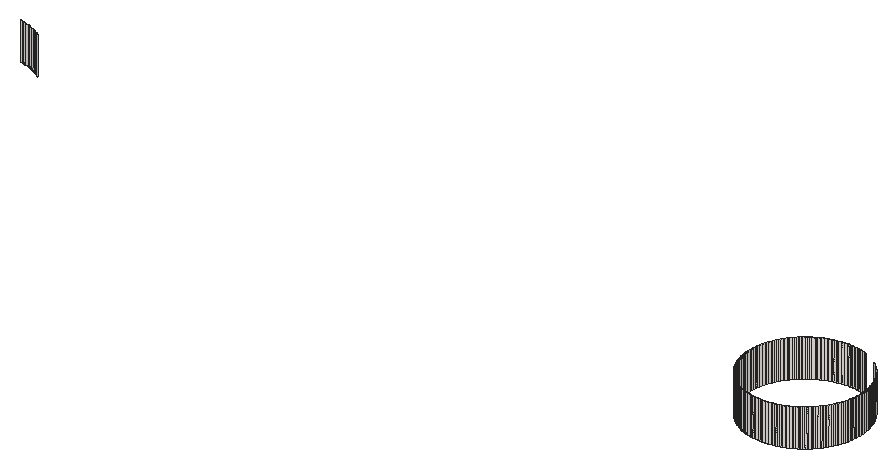
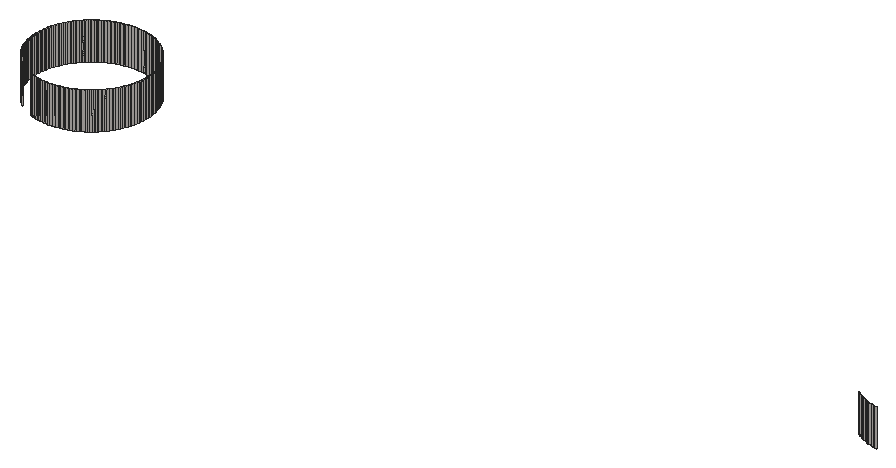
# SketchUp Ruby script. Lengths in inches.
U = 1.inch
M = Sketchup.active_model
def pt(a) = Geom::Point3d.new(a.map { |v| v * U })
def face(e, loops, mat)
  f = e.add_face(loops[0].map { |a| pt(a) })
  loops[1..].each { |l| e.add_face(l.map { |a| pt(a) }).erase! }
  f.material = f.back_material = mat if mat
  f
end
# faces: each face lists its corners as indices into pts; further lists are holes
def faces(e, pts, list, mat = nil) = list.each { |f| face(e, (f[0].is_a?(Array) ? f : [f]).map { |l| l.map { |i| pts[i] } }, mat) }
# xy, xz, yz: faces in a plane at the given z, y or x. An outline is a flat list of corners, or four numbers for a rectangle; further outlines are holes
def ring(l) = l.size == 4 ? [[l[0], l[1]], [l[2], l[1]], [l[2], l[3]], [l[0], l[3]]] : l.each_slice(2).to_a
def flat(e, list, mat, &to3) = list.each { |f| face(e, (f[0].is_a?(Array) ? f : [f]).map { |l| ring(l).map { |u, v| to3.(u, v) } }, mat) }
def xy(e, z, list, mat = nil) = flat(e, list, mat) { |x, y| [x, y, z] }
def xz(e, y, list, mat = nil) = flat(e, list, mat) { |x, z| [x, y, z] }
def yz(e, x, list, mat = nil) = flat(e, list, mat) { |y, z| [x, y, z] }
def lines(e, pts, list) = list.each { |a, b| e.add_line(pt(pts[a]), pt(pts[b])) }
# prism: a flat outline (further loops are holes) pulled along v
def prism(e, loops, v, mat = nil)
  f = face(e, loops, mat); d = Geom::Vector3d.new(v.map { |x| x * U })
  f.pushpull(f.normal.samedirection?(d) ? d.length : -d.length)
end
def box(e, o, s, mat = nil) = prism(e, [[o, [o[0] + s[0], o[1], o[2]], [o[0] + s[0], o[1] + s[1], o[2]], [o[0], o[1] + s[1], o[2]]]], [0, 0, s[2]], mat)
def at(x, y, z, deg = 0) = Geom::Transformation.translation(pt([x, y, z])) * Geom::Transformation.rotation(ORIGIN, Z_AXIS, deg.degrees)
def axes(o, x, y, z) = Geom::Transformation.new([*x, 0, *y, 0, *z, 0, *pt(o).to_a, 1])
def part(name) = M.definitions.add(name)
# library, detail: a bought-in or finely detailed component or shape, given as its bounding box
def library(name, o, s) = part(name).tap { |d| box(d.entities, o, s) }
def detail(e, o, s) = box(e.add_group.entities, o, s)
def put(e, d, t, mat = nil) = e.add_instance(d, t).tap { |i| i.material = mat if mat }
def group(e, t, mat = nil) = e.add_group.tap { |g| g.transformation = t; g.material = mat if mat }.entities
root = M.entities
M.materials.add("0001 AP 9436 AIR BREEZE").color = [243, 237, 232]
xz(root,40.5,[[68.91,106,68.98,108],[68.98,106,69.0625,108],[69.0625,106,69.14,108]],"0001 AP 9436 AIR BREEZE")
xz(root,40.51,[[68.75,106,68.83,108],[69.22,106,69.3,108]],"0001 AP 9436 AIR BREEZE")
xz(root,46.49,[[68.7,106,68.78,108],[69.17,106,69.25,108]],"0001 AP 9436 AIR BREEZE")
xz(root,46.5,[[68.86,106,68.9375,108],[68.9375,106,69.02,108],[69.02,106,69.09,108]],"0001 AP 9436 AIR BREEZE")
yz(root,66,[[43.36,106,43.4375,108],[43.4375,106,43.52,108],[43.52,106,43.59,108]],"0001 AP 9436 AIR BREEZE")
yz(root,66.01,[[43.2,106,43.28,108],[43.67,106,43.75,108]],"0001 AP 9436 AIR BREEZE")
yz(root,71.99,[[43.25,106,43.33,108],[43.72,106,43.8,108]],"0001 AP 9436 AIR BREEZE")
yz(root,72,[[43.41,106,43.48,108],[43.48,106,43.5625,108],[43.5625,106,43.64,108]],"0001 AP 9436 AIR BREEZE")
p = [[68.51,40.54,106],[68.4375,40.55,106],[68.4375,40.55,108],[68.51,40.54,108],[68.59,40.53,106],[68.59,40.53,108],
  [68.67,40.52,106],[68.67,40.52,108],[68.75,40.51,106],[68.75,40.51,108],[68.91,40.5,106],[68.83,40.51,106],
  [68.83,40.51,108],[68.91,40.5,108],[69.22,40.51,106],[69.14,40.5,106],[69.14,40.5,108],[69.22,40.51,108],
  [69.375,40.52,106],[69.3,40.51,106],[69.3,40.51,108],[69.375,40.52,108],[69.45,40.53,106],[69.45,40.53,108],
  [69.61,40.5625,106],[69.53,40.55,106],[69.53,40.55,108],[69.61,40.5625,108],[68.21,40.61,106],[68.13,40.63,106],
  [68.13,40.63,108],[68.21,40.61,108],[68.06,40.65,106],[68.06,40.65,108],[68.28,40.59,106],[68.28,40.59,108],
  [68.36,40.57,106],[68.36,40.57,108],[69.68,40.58,106],[69.68,40.58,108],[69.76,40.6,106],[69.76,40.6,108],
  [69.91,40.64,106],[69.84,40.62,106],[69.84,40.62,108],[69.91,40.64,108],[69.99,40.67,106],[69.99,40.67,108],
  [67.91,40.71,106],[67.84,40.73,106],[67.84,40.73,108],[67.91,40.71,108],[67.76,40.77,106],[67.76,40.77,108],
  [67.98,40.68,106],[67.98,40.68,108],[70.06,40.69,106],[70.06,40.69,108],[70.21,40.75,106],[70.13,40.72,106],
  [70.13,40.72,108],[70.21,40.75,108],[67.69,40.8,106],[67.625,40.83,106],[67.625,40.83,108],[67.69,40.8,108],
  [67.55,40.87,106],[67.55,40.87,108],[70.28,40.79,106],[70.28,40.79,108],[70.42,40.86,106],[70.35,40.82,106],
  [70.35,40.82,108],[70.42,40.86,108],[67.49,40.91,106],[67.42,40.95,106],[67.42,40.95,108],[67.49,40.91,108],
  [70.49,40.89,106],[70.49,40.89,108],[70.55,40.93,106],[70.55,40.93,108],[70.62,40.98,106],[70.62,40.98,108],
  [67.29,41.04,106],[67.22,41.08,106],[67.22,41.08,108],[67.29,41.04,108],[67.35,40.99,106],[67.35,40.99,108],
  [70.6875,41.02,106],[70.6875,41.02,108],[70.75,41.0625,106],[70.75,41.0625,108],[67.16,41.13,106],[67.1,41.18,106],
  [67.1,41.18,108],[67.16,41.13,108],[70.875,41.16,106],[70.8125,41.11,106],[70.8125,41.11,108],[70.875,41.16,108],
  [67.04,41.23,106],[67.04,41.23,108],[66.98,41.28,106],[66.98,41.28,108],[71,41.26,106],[70.9375,41.21,106],
  [70.9375,41.21,108],[71,41.26,108],[66.92,41.34,106],[66.92,41.34,108],[66.87,41.39,106],[66.87,41.39,108],
  [71.05,41.3125,106],[71.05,41.3125,108],[71.11,41.37,106],[71.11,41.37,108],[66.8125,41.45,106],[66.8125,41.45,108],
  [66.76,41.5,106],[66.76,41.5,108],[71.16,41.42,106],[71.16,41.42,108],[71.22,41.48,106],[71.22,41.48,108],
  [66.71,41.5625,106],[66.71,41.5625,108],[71.27,41.54,106],[71.27,41.54,108],[71.32,41.6,106],[71.32,41.6,108],
  [66.66,41.625,106],[66.61,41.6875,106],[66.61,41.6875,108],[66.66,41.625,108],[71.37,41.66,106],[71.37,41.66,108],
  [66.5625,41.75,106],[66.52,41.8125,106],[66.52,41.8125,108],[66.5625,41.75,108],[71.46,41.79,106],[71.42,41.72,106],
  [71.42,41.72,108],[71.46,41.79,108],[66.48,41.88,106],[66.48,41.88,108],[71.51,41.85,106],[71.51,41.85,108],
  [66.43,41.95,106],[66.43,41.95,108],[66.39,42.01,106],[66.39,42.01,108],[71.59,41.99,106],[71.55,41.92,106],
  [71.55,41.92,108],[71.59,41.99,108],[66.36,42.08,106],[66.36,42.08,108],[71.63,42.05,106],[71.63,42.05,108],
  [66.32,42.15,106],[66.32,42.15,108],[71.67,42.125,106],[71.67,42.125,108],[71.7,42.19,106],[71.7,42.19,108],
  [66.29,42.22,106],[66.29,42.22,108],[66.25,42.29,106],[66.25,42.29,108],[71.73,42.26,106],[71.73,42.26,108],
  [66.22,42.37,106],[66.22,42.37,108],[71.77,42.34,106],[71.77,42.34,108],[71.79,42.41,106],[71.79,42.41,108],
  [66.19,42.44,106],[66.19,42.44,108],[66.17,42.51,106],[66.17,42.51,108],[71.82,42.48,106],[71.82,42.48,108],
  [66.14,42.59,106],[66.14,42.59,108],[71.85,42.56,106],[71.85,42.56,108],[66.12,42.66,106],[66.12,42.66,108],
  [71.87,42.63,106],[71.87,42.63,108],[71.89,42.71,106],[71.89,42.71,108],[66.1,42.74,106],[66.1,42.74,108],
  [66.08,42.82,106],[66.08,42.82,108],[71.91,42.78,106],[71.91,42.78,108],[66.0625,42.89,106],[66.0625,42.89,108],
  [71.93,42.86,106],[71.93,42.86,108],[66.05,42.97,106],[66.05,42.97,108],[71.96,43.01,106],[71.95,42.9375,106],
  [71.95,42.9375,108],[71.96,43.01,108],[66.03,43.05,106],[66.03,43.05,108],[66.02,43.125,106],[66.02,43.125,108],
  [71.97,43.09,106],[71.97,43.09,108],[66.01,43.2,106],[66.01,43.2,108],[71.98,43.17,106],[71.98,43.17,108],
  [71.99,43.25,106],[71.99,43.25,108],[66.01,43.28,106],[66,43.36,106],[66,43.36,108],[66.01,43.28,108],
  [72,43.41,106],[71.99,43.33,106],[71.99,43.33,108],[72,43.41,108],[66,43.59,106],[66.01,43.67,106],
  [66.01,43.67,108],[66,43.59,108],[71.99,43.72,106],[72,43.64,106],[72,43.64,108],[71.99,43.72,108],
  [66.01,43.75,106],[66.02,43.83,106],[66.02,43.83,108],[66.01,43.75,108],[66.03,43.91,106],[66.03,43.91,108],
  [71.98,43.875,106],[71.99,43.8,106],[71.99,43.8,108],[71.98,43.875,108],[66.04,43.99,106],[66.04,43.99,108],
  [71.97,43.95,106],[71.97,43.95,108],[66.05,44.0625,106],[66.05,44.0625,108],[71.9375,44.11,106],[71.95,44.03,106],
  [71.95,44.03,108],[71.9375,44.11,108],[66.07,44.14,106],[66.07,44.14,108],[66.09,44.22,106],[66.09,44.22,108],
  [71.92,44.18,106],[71.92,44.18,108],[66.11,44.29,106],[66.11,44.29,108],[71.9,44.26,106],[71.9,44.26,108],
  [66.13,44.37,106],[66.13,44.37,108],[71.86,44.41,106],[71.88,44.34,106],[71.88,44.34,108],[71.86,44.41,108],
  [66.15,44.44,106],[66.15,44.44,108],[66.18,44.52,106],[66.18,44.52,108],[71.83,44.49,106],[71.83,44.49,108],
  [66.21,44.59,106],[66.21,44.59,108],[71.81,44.56,106],[71.81,44.56,108],[66.23,44.66,106],[66.23,44.66,108],
  [71.75,44.71,106],[71.78,44.63,106],[71.78,44.63,108],[71.75,44.71,108],[66.27,44.74,106],[66.27,44.74,108],
  [66.3,44.81,106],[66.3,44.81,108],[71.71,44.78,106],[71.71,44.78,108],[66.33,44.875,106],[66.33,44.875,108],
  [71.64,44.92,106],[71.68,44.85,106],[71.68,44.85,108],[71.64,44.92,108],[66.37,44.95,106],[66.37,44.95,108],
  [66.41,45.01,106],[66.41,45.01,108],[71.61,44.99,106],[71.61,44.99,108],[66.45,45.08,106],[66.45,45.08,108],
  [71.57,45.05,106],[71.57,45.05,108],[66.49,45.15,106],[66.49,45.15,108],[66.54,45.21,106],[66.54,45.21,108],
  [71.48,45.1875,106],[71.52,45.12,106],[71.52,45.12,108],[71.48,45.1875,108],[66.58,45.28,106],[66.58,45.28,108],
  [71.4375,45.25,106],[71.4375,45.25,108],[66.63,45.34,106],[66.63,45.34,108],[66.68,45.4,106],[66.68,45.4,108],
  [71.34,45.375,106],[71.39,45.3125,106],[71.39,45.3125,108],[71.34,45.375,108],[66.73,45.46,106],[66.73,45.46,108],
  [71.24,45.5,106],[71.29,45.4375,106],[71.29,45.4375,108],[71.24,45.5,108],[66.78,45.52,106],[66.78,45.52,108],
  [66.84,45.58,106],[66.84,45.58,108],[71.1875,45.55,106],[71.1875,45.55,108],[66.89,45.63,106],[66.89,45.63,108],
  [66.95,45.6875,106],[66.95,45.6875,108],[71.08,45.66,106],[71.13,45.61,106],[71.13,45.61,108],[71.08,45.66,108],
  [67,45.74,106],[67,45.74,108],[67.0625,45.79,106],[67.0625,45.79,108],[70.96,45.77,106],[71.02,45.72,106],
  [71.02,45.72,108],[70.96,45.77,108],[67.125,45.84,106],[67.125,45.84,108],[67.1875,45.89,106],[67.1875,45.89,108],
  [70.84,45.87,106],[70.9,45.82,106],[70.9,45.82,108],[70.84,45.87,108],[25.71,45.96,106],[25.78,45.92,106],
  [25.78,45.92,108],[25.71,45.96,108],[67.25,45.9375,106],[67.25,45.9375,108],[67.3125,45.98,106],[67.3125,45.98,108],
  [70.78,45.92,106],[70.78,45.92,108],[25.51,46.09,106],[25.58,46.05,106],[25.58,46.05,108],[25.51,46.09,108],
  [25.65,46.01,106],[25.65,46.01,108],[67.38,46.02,106],[67.38,46.02,108],[67.45,46.07,106],[67.45,46.07,108],
  [25.375,46.17,106],[25.45,46.13,106],[25.45,46.13,108],[25.375,46.17,108],[67.51,46.11,106],[67.51,46.11,108],
  [67.58,46.14,106],[67.58,46.14,108],[67.65,46.18,106],[67.65,46.18,108],[25.16,46.27,106],[25.24,46.23,106],
  [25.24,46.23,108],[25.16,46.27,108],[25.31,46.2,106],[25.31,46.2,108],[67.72,46.21,106],[67.72,46.21,108],
  [67.79,46.25,106],[67.79,46.25,108],[67.87,46.28,106],[67.87,46.28,108],[24.87,46.37,106],[24.94,46.35,106],
  [24.94,46.35,108],[24.87,46.37,108],[25.02,46.32,106],[25.02,46.32,108],[25.09,46.29,106],[25.09,46.29,108],
  [67.94,46.31,106],[67.94,46.31,108],[68.01,46.33,106],[68.01,46.33,108],[68.09,46.36,106],[68.09,46.36,108],
  [69.87,46.37,106],[69.94,46.35,106],[69.94,46.35,108],[69.87,46.37,108],[70.02,46.32,106],[70.02,46.32,108],
  [24.49,46.46,106],[24.5625,46.45,106],[24.5625,46.45,108],[24.49,46.46,108],[24.64,46.43,106],[24.64,46.43,108],
  [24.72,46.41,106],[24.72,46.41,108],[24.79,46.39,106],[24.79,46.39,108],[68.16,46.38,106],[68.16,46.38,108],
  [68.24,46.4,106],[68.24,46.4,108],[68.32,46.42,106],[68.32,46.42,108],[68.39,46.4375,106],[68.39,46.4375,108],
  [68.47,46.45,106],[68.47,46.45,108],[69.49,46.46,106],[69.5625,46.45,106],[69.5625,46.45,108],[69.49,46.46,108],
  [69.64,46.43,106],[69.64,46.43,108],[69.72,46.41,106],[69.72,46.41,108],[69.79,46.39,106],[69.79,46.39,108],
  [24.41,46.47,106],[24.41,46.47,108],[68.55,46.47,106],[68.55,46.47,108],[68.625,46.48,106],[68.625,46.48,108],
  [68.7,46.49,106],[68.7,46.49,108],[68.78,46.49,106],[68.86,46.5,106],[68.86,46.5,108],[68.78,46.49,108],
  [69.09,46.5,106],[69.17,46.49,106],[69.17,46.49,108],[69.09,46.5,108],[69.25,46.49,106],[69.33,46.48,106],
  [69.33,46.48,108],[69.25,46.49,108],[69.41,46.47,106],[69.41,46.47,108]]
faces(root,p,[[0,1,2,3],[4,0,3,5],[6,4,5,7],[8,6,7,9],[10,11,12,13],[14,15,16,17],[18,19,20,21],[22,18,21,23],
  [24,25,26,27],[25,22,23,26],[28,29,30,31],[29,32,33,30],[34,28,31,35],[36,34,35,37],[1,36,37,2],[38,24,27,39],
  [40,38,39,41],[42,43,44,45],[43,40,41,44],[46,42,45,47],[48,49,50,51],[49,52,53,50],[54,48,51,55],[32,54,55,33],
  [56,46,47,57],[58,59,60,61],[59,56,57,60],[62,63,64,65],[63,66,67,64],[52,62,65,53],[68,58,61,69],[70,71,72,73],
  [71,68,69,72],[74,75,76,77],[66,74,77,67],[78,70,73,79],[80,78,79,81],[82,80,81,83],[84,85,86,87],[88,84,87,89],
  [75,88,89,76],[90,82,83,91],[92,90,91,93],[94,95,96,97],[85,94,97,86],[98,99,100,101],[99,92,93,100],[95,102,103,96],
  [102,104,105,103],[106,107,108,109],[107,98,101,108],[104,110,111,105],[110,112,113,111],[114,106,109,115],[116,114,115,117],[112,118,119,113],
  [118,120,121,119],[122,116,117,123],[124,122,123,125],[120,126,127,121],[128,124,125,129],[130,128,129,131],[132,133,134,135],[126,132,135,127],
  [136,130,131,137],[138,139,140,141],[133,138,141,134],[142,143,144,145],[143,136,137,144],[139,146,147,140],[148,142,145,149],[146,150,151,147],
  [150,152,153,151],[154,155,156,157],[155,148,149,156],[152,158,159,153],[160,154,157,161],[158,162,163,159],[164,160,161,165],[166,164,165,167],
  [162,168,169,163],[168,170,171,169],[172,166,167,173],[170,174,175,171],[176,172,173,177],[178,176,177,179],[174,180,181,175],[180,182,183,181],
  [184,178,179,185],[182,186,187,183],[188,184,185,189],[186,190,191,187],[192,188,189,193],[194,192,193,195],[190,196,197,191],[196,198,199,197],
  [200,194,195,201],[198,202,203,199],[204,200,201,205],[202,206,207,203],[208,209,210,211],[209,204,205,210],[206,212,213,207],[212,214,215,213],
  [216,208,211,217],[214,218,219,215],[220,216,217,221],[222,220,221,223],[224,225,226,227],[228,229,230,231],[232,233,234,235],[236,237,238,239],
  [240,241,242,243],[241,244,245,242],[246,247,248,249],[244,250,251,245],[252,246,249,253],[250,254,255,251],[256,257,258,259],[257,252,253,258],
  [254,260,261,255],[260,262,263,261],[264,256,259,265],[262,266,267,263],[268,264,265,269],[266,270,271,267],[272,273,274,275],[273,268,269,274],
  [270,276,277,271],[276,278,279,277],[280,272,275,281],[278,282,283,279],[284,280,281,285],[282,286,287,283],[288,289,290,291],[289,284,285,290],
  [286,292,293,287],[292,294,295,293],[296,288,291,297],[294,298,299,295],[300,301,302,303],[301,296,297,302],[298,304,305,299],[304,306,307,305],
  [308,300,303,309],[306,310,311,307],[312,308,309,313],[310,314,315,311],[314,316,317,315],[318,319,320,321],[319,312,313,320],[316,322,323,317],
  [324,318,321,325],[322,326,327,323],[326,328,329,327],[330,331,332,333],[331,324,325,332],[328,334,335,329],[336,337,338,339],[337,330,333,338],
  [334,340,341,335],[340,342,343,341],[344,336,339,345],[342,346,347,343],[346,348,349,347],[350,351,352,353],[351,344,345,352],[348,354,355,349],
  [354,356,357,355],[358,359,360,361],[359,350,353,360],[356,362,363,357],[362,364,365,363],[366,367,368,369],[367,358,361,368],[370,371,372,373],
  [364,374,375,365],[374,376,377,375],[378,366,369,379],[380,381,382,383],[381,384,385,382],[384,370,373,385],[376,386,387,377],[386,388,389,387],
  [390,391,392,393],[391,380,383,392],[388,394,395,389],[394,396,397,395],[396,398,399,397],[400,401,402,403],[401,404,405,402],[404,390,393,405],
  [398,406,407,399],[406,408,409,407],[408,410,411,409],[412,413,414,415],[413,416,417,414],[416,418,419,417],[418,400,403,419],[410,420,421,411],
  [420,422,423,421],[422,424,425,423],[426,427,428,429],[427,430,431,428],[432,433,434,435],[433,436,437,434],[436,438,439,437],[438,440,441,439],
  [440,412,415,441],[424,442,443,425],[442,444,445,443],[444,446,447,445],[446,448,449,447],[448,450,451,449],[452,453,454,455],[453,456,457,454],
  [456,458,459,457],[458,460,461,459],[460,426,429,461],[462,432,435,463],[450,464,465,451],[464,466,467,465],[466,468,469,467],[470,471,472,473],
  [474,475,476,477],[478,479,480,481],[479,482,483,480],[482,452,455,483]],"0001 AP 9436 AIR BREEZE")
